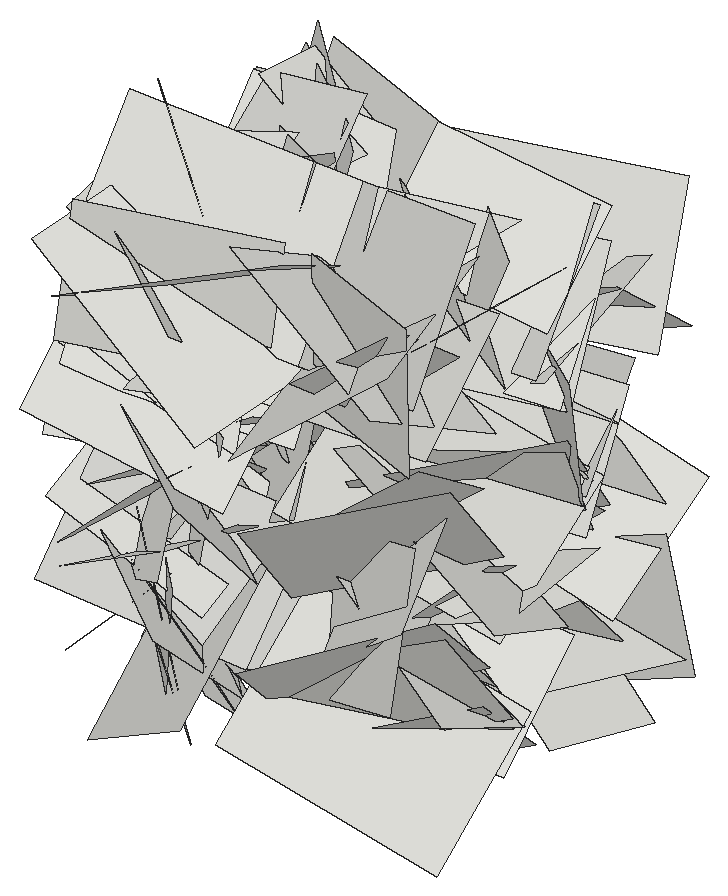
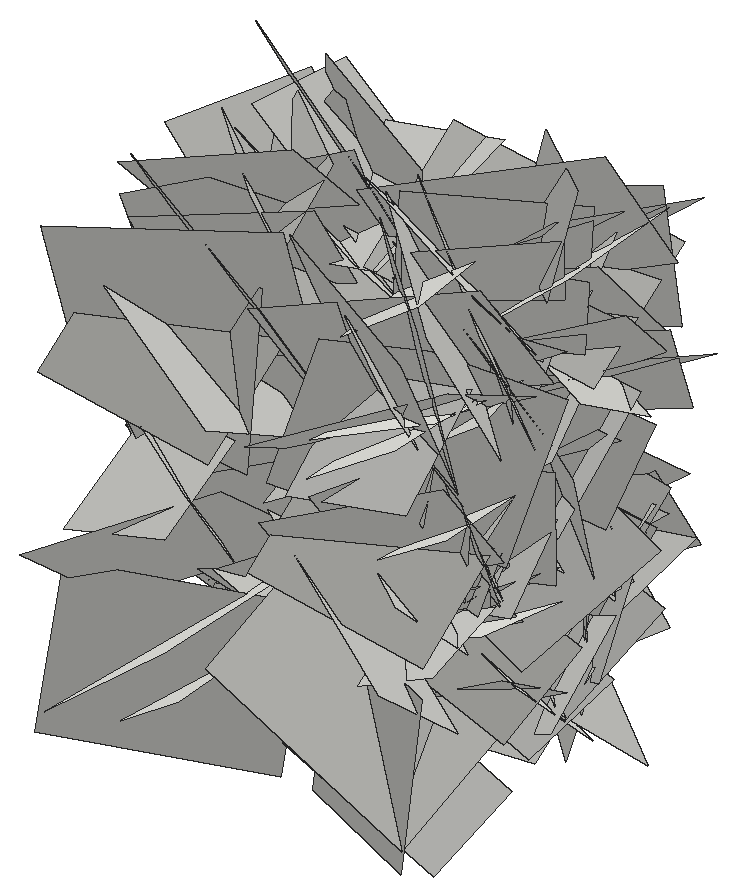
# SketchUp Ruby script. Lengths in inches.
U = 1.inch
M = Sketchup.active_model
def pt(a) = Geom::Point3d.new(a.map { |v| v * U })
def face(e, loops, mat)
  f = e.add_face(loops[0].map { |a| pt(a) })
  loops[1..].each { |l| e.add_face(l.map { |a| pt(a) }).erase! }
  f.material = f.back_material = mat if mat
  f
end
# faces: each face lists its corners as indices into pts; further lists are holes
def faces(e, pts, list, mat = nil) = list.each { |f| face(e, (f[0].is_a?(Array) ? f : [f]).map { |l| l.map { |i| pts[i] } }, mat) }
# xy, xz, yz: faces in a plane at the given z, y or x. An outline is a flat list of corners, or four numbers for a rectangle; further outlines are holes
def ring(l) = l.size == 4 ? [[l[0], l[1]], [l[2], l[1]], [l[2], l[3]], [l[0], l[3]]] : l.each_slice(2).to_a
def flat(e, list, mat, &to3) = list.each { |f| face(e, (f[0].is_a?(Array) ? f : [f]).map { |l| ring(l).map { |u, v| to3.(u, v) } }, mat) }
def xy(e, z, list, mat = nil) = flat(e, list, mat) { |x, y| [x, y, z] }
def xz(e, y, list, mat = nil) = flat(e, list, mat) { |x, z| [x, y, z] }
def yz(e, x, list, mat = nil) = flat(e, list, mat) { |y, z| [x, y, z] }
def lines(e, pts, list) = list.each { |a, b| e.add_line(pt(pts[a]), pt(pts[b])) }
# prism: a flat outline (further loops are holes) pulled along v
def prism(e, loops, v, mat = nil)
  f = face(e, loops, mat); d = Geom::Vector3d.new(v.map { |x| x * U })
  f.pushpull(f.normal.samedirection?(d) ? d.length : -d.length)
end
def box(e, o, s, mat = nil) = prism(e, [[o, [o[0] + s[0], o[1], o[2]], [o[0] + s[0], o[1] + s[1], o[2]], [o[0], o[1] + s[1], o[2]]]], [0, 0, s[2]], mat)
def at(x, y, z, deg = 0) = Geom::Transformation.translation(pt([x, y, z])) * Geom::Transformation.rotation(ORIGIN, Z_AXIS, deg.degrees)
def axes(o, x, y, z) = Geom::Transformation.new([*x, 0, *y, 0, *z, 0, *pt(o).to_a, 1])
def part(name) = M.definitions.add(name)
# library, detail: a bought-in or finely detailed component or shape, given as its bounding box
def library(name, o, s) = part(name).tap { |d| box(d.entities, o, s) }
def detail(e, o, s) = box(e.add_group.entities, o, s)
def put(e, d, t, mat = nil) = e.add_instance(d, t).tap { |i| i.material = mat if mat }
def group(e, t, mat = nil) = e.add_group.tap { |g| g.transformation = t; g.material = mat if mat }.entities
root = M.entities
c1 = part("Component\#6")
p = [[0.01,0,0],[0,3.24,4.54],[4.32,3.24,4.54],[4.33,0,0]]
faces(c1.entities,p,[[0,1,2,3]])
put(root,c1,axes([24.34,164.95,29.96],[-0.04265,0.57286,-0.52342],[0.15347,-0.50938,-0.56862],[0.80809,0.12697,0.08036]))
put(root,c1,axes([24.34,167.51,23.32],[-0.04127,-0.8056,0.43064],[-0.05085,0.43224,0.80425],[0.96695,-0.01165,0.06068]))
put(root,c1,axes([24.34,163.99,40.83],[0.08038,0.23372,-0.81219],[-0.10222,-0.80774,-0.24144],[0.89001,-0.11388,0.04562]))
put(root,c1,axes([24.34,164.8,26.41],[0.06555,-0.88967,-0.10275],[-0.1194,-0.1099,0.88381],[0.94178,0.04799,0.1192]))
put(root,c1,axes([28.31,169.82,24.93],[-0.00586,-0.68753,0.27068],[-0.05817,0.27032,0.6855],[-0.78107,-0.01497,-0.05308]))
put(root,c1,axes([28.31,164.96,33.58],[-0.03363,-0.67551,-0.53197],[0.14584,-0.52946,0.66412],[-0.89967,-0.06058,0.12754]))
put(root,c1,axes([24.34,168.875,35.8],[0.07444,0.7996,-0.0855],[0.00091,-0.0859,-0.80263],[0.85241,-0.06974,0.00832]))
put(root,c1,axes([24.34,164.5,23.79],[0.04443,0.667,0.37408],[0.11412,0.36576,-0.66423],[0.80255,-0.08894,0.07374]))
put(root,c1,axes([24.34,162.92,24.26],[0.16568,0.16434,-0.80239],[-0.1251,-0.80382,-0.18763],[0.85913,-0.14874,0.12742]))
put(root,c1,axes([24.34,162.61,28.57],[-0.04222,-0.49534,0.62953],[0.20196,0.60636,0.48917],[0.82474,-0.17384,-0.08755]))
put(root,c1,axes([24.34,162.43,26.35],[0.02315,-0.70596,0.51236],[-0.01203,0.51225,0.70629],[0.92456,0.02434,-0.00364]))
put(root,c1,axes([28.31,171.89,34.33],[0.10287,-0.74562,-0.1631],[-0.15609,-0.17961,0.73351],[-0.79385,-0.06131,-0.16536]))
put(root,c1,axes([24.34,171.21,38.93],[-0.24063,-0.51313,-1.11059],[-0.16085,-1.10901,0.54342],[1.28679,-0.23458,-0.13976]))
put(root,c1,axes([24.34,166.53,31.68],[-0.02185,0.89564,-0.0065],[0.05171,-0.00537,-0.89456],[0.948,0.02094,0.04865]))
put(root,c1,axes([24.34,158.45,30.92],[-0.16236,0.46297,0.88251],[0.09478,0.89566,-0.45434],[1.05211,-0.00924,0.17712]))
put(root,c1,axes([24.34,163.85,33.45],[-0.03445,-0.73428,-0.4148],[0.17499,-0.41262,0.71747],[0.87664,0.05351,-0.15952]))
put(root,c1,axes([28.31,168.18,25.35],[-0.0356,-0.79141,-0.13903],[0.13499,-0.14264,0.78117],[-0.84098,0.01061,0.13127]))
put(root,c1,axes([28.31,167.69,34.89],[-0.01272,-0.59445,-0.3878],[-0.01652,-0.38754,0.59453],[-0.75216,0.01856,-0.0065]))
put(root,c1,axes([24.34,171.77,39.47],[-0.25632,-0.1505,-1.28885],[-0.2021,-1.29268,0.18672],[1.36053,-0.22038,-0.21508]))
put(root,c1,axes([24.34,166.33,22.3],[-0.05809,-0.87115,0.26873],[0.09257,0.26296,0.87026],[0.96191,-0.07791,-0.06752]))
put(root,c1,axes([24.34,162.32,28.44],[0.12821,-0.42216,-0.69512],[-0.01339,-0.70366,0.42514],[0.86197,0.05186,0.11]))
put(root,c1,axes([28.31,169.92,30.86],[-0.08798,0.07784,-0.70174],[0.08853,-0.70052,-0.08758],[-0.74315,-0.09267,0.07264]))
put(root,c1,axes([24.34,164.2,31.01],[-0.06613,-0.18181,-0.96198],[0.02897,-0.96387,0.1804],[1.03734,0.01533,-0.06637]))
put(root,c1,axes([24.34,161.79,25.53],[0.01152,-0.82607,0.19056],[0.15176,0.18963,0.81386],[0.88572,-0.02175,-0.14193]))
put(root,c1,axes([28.31,169.17,27.35],[-0.00515,-0.4485,-0.48712],[-0.04455,-0.48594,0.44784],[-0.70046,0.0342,-0.02491]))
put(root,c1,axes([28.31,158.39,26.84],[0.02686,0.84806,0.10272],[0.17857,0.09579,-0.83237],[-0.88773,0.04493,-0.16432]))
put(root,c1,axes([28.31,159.67,28.14],[0.12868,0.67272,0.52517],[0.08613,0.51893,-0.68352],[-0.90053,0.14576,0.00967]))
put(root,c1,axes([28.31,160.06,22.6],[0.02839,-0.24478,0.77995],[0.15528,0.76918,0.23637],[-0.85248,0.13195,0.06903]))
put(root,c1,axes([28.31,159.46,22.85],[0.09982,-0.0635,0.89488],[0.1784,0.88507,0.04509],[-0.93408,0.16225,0.10424]))
put(root,c1,axes([28.31,168.82,35.84],[-0.04533,0.37689,0.51175],[0.01637,0.51337,-0.3768],[-0.67349,-0.01289,-0.04361]))
put(root,c1,axes([24.34,157.3125,32.29],[-0.25179,1.05256,0.51222],[0.06429,0.53303,-1.06718],[1.23914,0.18623,0.15945]))
put(root,c1,axes([24.34,167.29,35.58],[0.17595,-0.29467,-0.74084],[0.05215,-0.7515,0.30993],[0.84352,0.10793,0.13537]))
put(root,c1,axes([28.31,171.91,32.4],[-0.07209,-0.36069,-0.54144],[0.07785,-0.54516,0.35394],[-0.6852,-0.024,0.09718]))
put(root,c1,axes([24.34,165.04,27.71],[-0.04822,0.07219,0.94774],[0.14201,0.93984,-0.06516],[0.99746,-0.13032,0.05509]))
put(root,c1,axes([28.31,162.33,29.83],[0.22776,0.38392,-0.75072],[-0.01782,-0.77261,-0.39993],[-0.89361,0.11326,-0.18337]))
put(root,c1,axes([28.31,168.23,31.98],[0.11552,-0.73847,0.10601],[-0.00435,0.10653,0.74638],[-0.79079,-0.10846,0.01138]))
put(root,c1,axes([28.31,158.35,30.49],[0.08461,0.81055,-0.03501],[0.12527,-0.04642,-0.80528],[-0.85081,0.07377,-0.12204]))
put(root,c1,axes([24.34,159.15,32.85],[-0.28722,0.93511,0.86971],[-0.00467,0.88838,-0.95656],[1.35365,0.20148,0.18123]))
put(root,c1,axes([28.31,170.38,37.22],[0.01844,-0.65259,0.06973],[0.0154,0.07012,0.65262],[-0.69551,-0.01575,0.0163]))
put(root,c1,axes([24.34,162.15,25.43],[-0.09766,0.84172,-0.54191],[0.18116,-0.52299,-0.84139],[1.04557,0.16923,0.09516]))
put(root,c1,axes([28.31,165.16,26.22],[-0.00662,-0.41647,0.48084],[0.04981,0.47925,0.41571],[-0.67246,0.0396,0.02606]))
put(root,c1,axes([28.31,166.74,28.03],[0.20581,0.5378,0.53941],[-0.0447,0.5634,-0.54654],[-0.80617,0.10606,0.16802]))
put(root,c1,axes([28.31,167.3,30.05],[0.09755,-0.36279,0.79394],[0.2327,0.7823,0.33203],[-0.89554,0.16375,0.17276]))
put(root,c1,axes([28.31,163.79,31.02],[0.0186,-0.39942,0.51021],[0.04828,0.50989,0.39761],[-0.68514,0.02509,0.04187]))
put(root,c1,axes([28.31,168.24,29.62],[0.00844,-0.1319,-0.59476],[0.00779,-0.59475,0.132],[-0.64572,-0.0089,-0.00618]))
put(root,c1,axes([24.34,168.37,37.02],[-0.06582,-0.55881,-0.84289],[0.17414,-0.83883,0.54402],[1.05774,0.10333,-0.14201]))
put(root,c1,axes([24.34,162.55,24.47],[0.08094,0.6993,-0.63815],[0.06519,-0.64254,-0.69674],[1.00139,-0.01469,0.09694]))
put(root,c1,axes([28.31,167.47,38.84],[0.19203,-0.25676,-0.78485],[0.09527,-0.79261,0.28005],[-0.87013,-0.14344,-0.14255]))
put(root,c1,axes([28.31,168.14,25.37],[0.00005,-0.54267,0.44601],[0.16088,0.43548,0.52984],[-0.72699,0.09633,0.11728]))
put(root,c1,axes([24.34,169.13,31.47],[0.22896,-0.22184,-0.76377],[0.12794,-0.77313,0.25869],[0.83329,0.17965,0.17014]))
put(root,c1,axes([24.34,164.67,22.86],[-0.07455,-1.03669,0.46758],[0.01691,0.46753,1.03897],[1.20537,-0.07068,0.01434]))
put(root,c1,axes([28.31,161.42,33.85],[0.12931,-0.58697,0.4315],[0.06321,0.44408,0.58723],[-0.76963,-0.06214,0.12073]))
put(root,c1,axes([24.34,160.7,27.63],[-0.09928,0.64406,-0.88513],[0.13228,-0.87629,-0.65083],[1.15276,0.15602,-0.00154]))
put(root,c1,axes([24.34,159.57,38.3125],[-0.19748,1.37219,0.09956],[-0.15298,0.08042,-1.37849],[1.4503,0.19533,-0.13185]))
put(root,c1,axes([28.31,165.91,24.52],[-0.03596,-0.58924,0.24858],[0.15481,0.23521,0.57749],[-0.65999,0.08727,0.12191]))
put(root,c1,axes([24.34,166.55,31.56],[0.0814,0.41102,-0.8284],[0.17089,-0.82447,-0.39413],[0.96524,0.11131,0.13964]))
put(root,c1,axes([28.31,169.1,21.1],[0.05323,-0.42134,0.48328],[0.06346,0.48572,0.41725],[-0.67666,0.01241,0.07715]))
put(root,c1,axes([24.34,166.67,25.47],[-0.29316,-1.18227,0.54308],[0.10516,0.53443,1.21398],[1.37509,-0.29293,0.02294]))
put(root,c1,axes([24.34,168.75,37.98],[-0.06882,-0.53698,-1.12739],[-0.1022,-1.12338,0.54063],[1.31971,-0.115,-0.01692]))
put(root,c1,axes([24.34,158.58,28.72],[0.17742,0.80309,0.64454],[-0.10421,0.66248,-0.79991],[1.08655,-0.0676,-0.18196]))
put(root,c1,axes([28.31,163.1,21.29],[0.03251,-0.459,0.52355],[0.17075,0.51451,0.44164],[-0.71801,0.10157,0.12873]))
put(root,c1,axes([24.34,169.04,36.23],[-0.04162,0.78981,-0.64322],[0.24351,-0.62024,-0.77563],[1.05189,0.17484,0.15411]))
put(root,c1,axes([24.34,170.89,20.28],[0.12274,-1.02279,0.17958],[-0.0333,0.17716,1.02926],[1.10024,0.11946,0.01112]))
put(root,c1,axes([24.34,167.53,29.6],[0.04916,0.6172,0.8297],[0.08211,0.82613,-0.61887],[1.09305,-0.08981,0.00917]))
put(root,c1,axes([24.34,171.44,27.64],[0.05126,-0.8571,0.56567],[0.11133,0.56746,0.85083],[1.08285,-0.01777,-0.11425]))
put(root,c1,axes([28.31,163.13,28.77],[0.13219,-0.55975,0.33448],[0.05965,0.34851,0.56225],[-0.68862,-0.07726,0.11291]))
put(root,c1,axes([24.34,163.625,35.04],[0.27654,-0.44632,0.88094],[-0.09901,0.89592,0.48157],[1.04211,0.20356,-0.18801]))
put(root,c1,axes([24.34,167.41,29.34],[-0.20833,-0.42173,1.22713],[0.0869,1.23461,0.43743],[1.37269,-0.14217,0.15855]))
put(root,c1,axes([24.34,168.84,39.14],[0.0295,-0.69575,-0.73723],[0.22295,-0.71749,0.68506],[1.05113,0.17171,-0.12461]))
put(root,c1,axes([24.34,163.85,26.9],[0.03329,1.04875,0.11229],[0.24045,0.10299,-1.02538],[1.09187,-0.05466,0.22238]))
put(root,c1,axes([24.34,160.22,28.4],[0.15479,0.80897,-0.76348],[-0.02106,-0.76802,-0.81757],[1.17891,-0.11994,0.08565]))
put(root,c1,axes([24.34,169.63,32.59],[0.01533,-0.4611,-1.03377],[0.17767,-1.02158,0.45801],[1.18663,0.15892,-0.05522]))
put(root,c1,axes([24.34,159.8,34.2],[-0.03301,0.77795,0.85676],[0.24326,0.8442,-0.75821],[1.20233,-0.14944,0.17692]))
put(root,c1,axes([24.34,166.97,25.06],[-0.03339,-0.82276,-0.77538],[0.30966,-0.75526,0.78954],[1.15769,0.17829,-0.23355]))
put(root,c1,axes([24.34,165.55,34.43],[-0.04885,1.13911,0.54464],[0.08516,0.54654,-1.13629],[1.33566,0.00681,0.09237]))
put(root,c1,axes([24.34,164.92,23.28],[0.02573,-1.02703,-0.88101],[-0.12942,-0.87922,1.02158],[1.42847,-0.06116,0.10843]))
put(root,c1,axes([24.34,160.96,32.62],[0.12215,0.75895,-0.88724],[0.014,-0.89234,-0.7616],[1.23753,-0.06482,0.09619]))
put(root,c1,axes([24.34,172.54,38.57],[-0.12011,-0.4932,-1.18141],[0.20578,-1.17893,0.47355],[1.34134,0.1367,-0.17844]))
put(root,c1,axes([24.34,171.44,26.6],[-0.03428,0.27698,-1.26013],[0.06702,-1.25867,-0.27828],[1.36598,0.0687,-0.01797]))
put(root,c1,axes([24.34,173.53,27.66],[0.08068,-0.97468,-0.75893],[0.01331,-0.75972,0.97695],[1.30935,0.06778,0.03684]))
put(root,c1,axes([24.34,158.99,33.95],[0.09747,0.08794,1.12692],[0.17247,1.11783,-0.1005],[1.18568,-0.16983,-0.07802]))
put(root,c1,axes([24.34,166.62,31.96],[0.21061,0.75098,-0.921],[-0.02022,-0.93165,-0.76377],[1.25951,-0.14053,0.14175]))
put(root,c1,axes([24.34,158.06,26.05],[0.19995,0.52409,1.06255],[0.00833,1.07535,-0.5318],[1.25583,-0.09057,-0.16565]))
put(root,c1,axes([24.34,172.42,21.79],[0.22827,-1.35966,0.24048],[-0.1567,0.21929,1.3722],[1.45519,0.2369,0.11004]))
put(root,c1,axes([24.34,165.11,34.6875],[0.03998,0.77126,1.05992],[0.2457,1.03973,-0.76482],[1.36759,-0.20934,0.10642]))
put(root,c1,axes([24.34,159.18,36.25],[0.04304,0.74935,1.15311],[0.14712,1.14549,-0.74928],[1.45028,-0.13844,0.04179]))
put(root,c1,axes([24.34,168.45,29.92],[0.2904,-0.81126,-1.09363],[-0.15157,-1.12651,0.79984],[1.4354,0.04517,0.30571]))
put(root,c1,axes([24.34,157.9,37.93],[0.24747,1.3445,0.30187],[-0.11522,0.32319,-1.35538],[1.4561,-0.20293,-0.15855]))
put(root,c1,axes([24.34,163.2,33.68],[0.16473,-1.2102,0.57798],[0.2383,0.59712,1.18983],[1.40149,0.04071,-0.27024]))
put(root,c1,axes([38.11,163.2,33.68],[-0.16473,-1.2102,0.57798],[-0.2383,0.59712,1.18983],[-1.40149,0.04071,-0.27024]))
put(root,c1,axes([38.11,157.9,37.93],[-0.24747,1.3445,0.30187],[0.11522,0.32319,-1.35538],[-1.4561,-0.20293,-0.15855]))
put(root,c1,axes([38.11,168.45,29.92],[-0.2904,-0.81126,-1.09363],[0.15157,-1.12651,0.79984],[-1.4354,0.04517,0.30571]))
put(root,c1,axes([38.11,159.18,36.25],[-0.04304,0.74935,1.15311],[-0.14712,1.14549,-0.74928],[-1.45028,-0.13844,0.04179]))
put(root,c1,axes([38.11,165.11,34.6875],[-0.03998,0.77126,1.05992],[-0.2457,1.03973,-0.76482],[-1.36759,-0.20934,0.10642]))
put(root,c1,axes([38.11,172.42,21.79],[-0.22827,-1.35966,0.24048],[0.1567,0.21929,1.3722],[-1.45519,0.2369,0.11004]))
put(root,c1,axes([38.11,158.06,26.05],[-0.19995,0.52409,1.06255],[-0.00833,1.07535,-0.5318],[-1.25583,-0.09057,-0.16565]))
put(root,c1,axes([38.11,166.62,31.96],[-0.21061,0.75098,-0.921],[0.02022,-0.93165,-0.76377],[-1.25951,-0.14053,0.14175]))
put(root,c1,axes([38.11,158.99,33.95],[-0.09747,0.08794,1.12692],[-0.17247,1.11783,-0.1005],[-1.18568,-0.16983,-0.07802]))
put(root,c1,axes([38.11,173.53,27.66],[-0.08068,-0.97468,-0.75893],[-0.01331,-0.75972,0.97695],[-1.30935,0.06778,0.03684]))
put(root,c1,axes([38.11,171.44,26.6],[0.03428,0.27698,-1.26013],[-0.06702,-1.25867,-0.27828],[-1.36598,0.0687,-0.01797]))
put(root,c1,axes([38.11,172.54,38.57],[0.12011,-0.4932,-1.18141],[-0.20578,-1.17893,0.47355],[-1.34134,0.1367,-0.17844]))
put(root,c1,axes([38.11,160.96,32.62],[-0.12215,0.75895,-0.88724],[-0.014,-0.89234,-0.7616],[-1.23753,-0.06482,0.09619]))
put(root,c1,axes([38.11,164.92,23.28],[-0.02573,-1.02703,-0.88101],[0.12942,-0.87922,1.02158],[-1.42847,-0.06116,0.10843]))
put(root,c1,axes([38.11,165.55,34.43],[0.04885,1.13911,0.54464],[-0.08516,0.54654,-1.13629],[-1.33566,0.00681,0.09237]))
put(root,c1,axes([38.11,166.97,25.06],[0.03339,-0.82276,-0.77538],[-0.30966,-0.75526,0.78954],[-1.15769,0.17829,-0.23355]))
put(root,c1,axes([38.11,159.8,34.2],[0.03301,0.77795,0.85676],[-0.24326,0.8442,-0.75821],[-1.20233,-0.14944,0.17692]))
put(root,c1,axes([38.11,169.63,32.59],[-0.01533,-0.4611,-1.03377],[-0.17767,-1.02158,0.45801],[-1.18663,0.15892,-0.05522]))
put(root,c1,axes([38.11,160.22,28.4],[-0.15479,0.80897,-0.76348],[0.02106,-0.76802,-0.81757],[-1.17891,-0.11994,0.08565]))
put(root,c1,axes([38.11,163.85,26.9],[-0.03329,1.04875,0.11229],[-0.24045,0.10299,-1.02538],[-1.09187,-0.05466,0.22238]))
put(root,c1,axes([38.11,168.84,39.14],[-0.0295,-0.69575,-0.73723],[-0.22295,-0.71749,0.68506],[-1.05113,0.17171,-0.12461]))
put(root,c1,axes([38.11,167.41,29.34],[0.20833,-0.42173,1.22713],[-0.0869,1.23461,0.43743],[-1.37269,-0.14217,0.15855]))
put(root,c1,axes([38.11,163.625,35.04],[-0.27654,-0.44632,0.88094],[0.09901,0.89592,0.48157],[-1.04211,0.20356,-0.18801]))
put(root,c1,axes([34.14,163.13,28.77],[-0.13219,-0.55975,0.33448],[-0.05965,0.34851,0.56225],[0.68862,-0.07726,0.11291]))
put(root,c1,axes([38.11,171.44,27.64],[-0.05126,-0.8571,0.56567],[-0.11133,0.56746,0.85083],[-1.08285,-0.01777,-0.11425]))
put(root,c1,axes([38.11,167.53,29.6],[-0.04916,0.6172,0.8297],[-0.08211,0.82613,-0.61887],[-1.09305,-0.08981,0.00917]))
put(root,c1,axes([38.11,170.89,20.28],[-0.12274,-1.02279,0.17958],[0.0333,0.17716,1.02926],[-1.10024,0.11946,0.01112]))
put(root,c1,axes([38.11,169.04,36.23],[0.04162,0.78981,-0.64322],[-0.24351,-0.62024,-0.77563],[-1.05189,0.17484,0.15411]))
put(root,c1,axes([34.14,163.1,21.29],[-0.03251,-0.459,0.52355],[-0.17075,0.51451,0.44164],[0.71801,0.10157,0.12873]))
put(root,c1,axes([38.11,158.58,28.72],[-0.17742,0.80309,0.64454],[0.10421,0.66248,-0.79991],[-1.08655,-0.0676,-0.18196]))
put(root,c1,axes([38.11,168.75,37.98],[0.06882,-0.53698,-1.12739],[0.1022,-1.12338,0.54063],[-1.31971,-0.115,-0.01692]))
put(root,c1,axes([38.11,166.67,25.47],[0.29316,-1.18227,0.54308],[-0.10516,0.53443,1.21398],[-1.37509,-0.29293,0.02294]))
put(root,c1,axes([34.14,169.1,21.1],[-0.05323,-0.42134,0.48328],[-0.06346,0.48572,0.41725],[0.67666,0.01241,0.07715]))
put(root,c1,axes([38.11,166.55,31.56],[-0.0814,0.41102,-0.8284],[-0.17089,-0.82447,-0.39413],[-0.96524,0.11131,0.13964]))
put(root,c1,axes([34.14,165.91,24.52],[0.03596,-0.58924,0.24858],[-0.15481,0.23521,0.57749],[0.65999,0.08727,0.12191]))
put(root,c1,axes([38.11,159.57,38.3125],[0.19748,1.37219,0.09956],[0.15298,0.08042,-1.37849],[-1.4503,0.19533,-0.13185]))
put(root,c1,axes([38.11,160.7,27.63],[0.09928,0.64406,-0.88513],[-0.13228,-0.87629,-0.65083],[-1.15276,0.15602,-0.00154]))
put(root,c1,axes([34.14,161.42,33.85],[-0.12931,-0.58697,0.4315],[-0.06321,0.44408,0.58723],[0.76963,-0.06214,0.12073]))
put(root,c1,axes([38.11,164.67,22.86],[0.07455,-1.03669,0.46758],[-0.01691,0.46753,1.03897],[-1.20537,-0.07068,0.01434]))
put(root,c1,axes([38.11,169.13,31.47],[-0.22896,-0.22184,-0.76377],[-0.12794,-0.77313,0.25869],[-0.83329,0.17965,0.17014]))
put(root,c1,axes([34.14,168.14,25.37],[-0.00005,-0.54267,0.44601],[-0.16088,0.43548,0.52984],[0.72699,0.09633,0.11728]))
put(root,c1,axes([34.14,167.47,38.84],[-0.19203,-0.25676,-0.78485],[-0.09527,-0.79261,0.28005],[0.87013,-0.14344,-0.14255]))
put(root,c1,axes([38.11,162.55,24.47],[-0.08094,0.6993,-0.63815],[-0.06519,-0.64254,-0.69674],[-1.00139,-0.01469,0.09694]))
put(root,c1,axes([38.11,168.37,37.02],[0.06582,-0.55881,-0.84289],[-0.17414,-0.83883,0.54402],[-1.05774,0.10333,-0.14201]))
